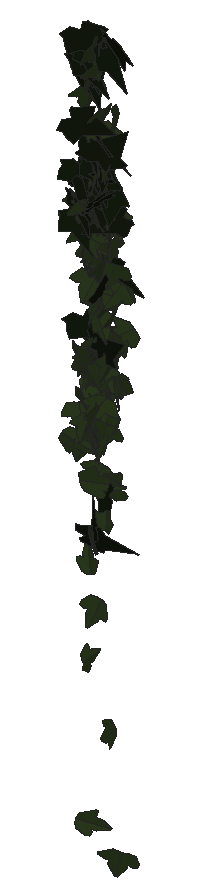
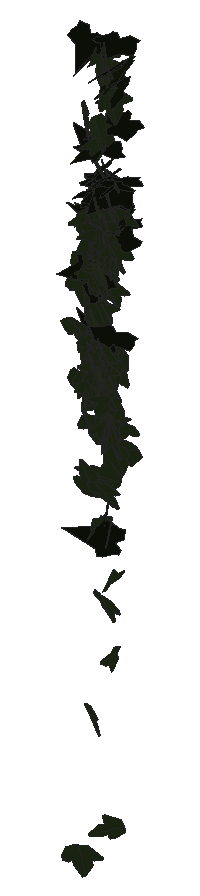
# SketchUp Ruby script. Lengths in inches.
U = 1.inch
M = Sketchup.active_model
def pt(a) = Geom::Point3d.new(a.map { |v| v * U })
def face(e, loops, mat)
  f = e.add_face(loops[0].map { |a| pt(a) })
  loops[1..].each { |l| e.add_face(l.map { |a| pt(a) }).erase! }
  f.material = f.back_material = mat if mat
  f
end
# faces: each face lists its corners as indices into pts; further lists are holes
def faces(e, pts, list, mat = nil) = list.each { |f| face(e, (f[0].is_a?(Array) ? f : [f]).map { |l| l.map { |i| pts[i] } }, mat) }
# xy, xz, yz: faces in a plane at the given z, y or x. An outline is a flat list of corners, or four numbers for a rectangle; further outlines are holes
def ring(l) = l.size == 4 ? [[l[0], l[1]], [l[2], l[1]], [l[2], l[3]], [l[0], l[3]]] : l.each_slice(2).to_a
def flat(e, list, mat, &to3) = list.each { |f| face(e, (f[0].is_a?(Array) ? f : [f]).map { |l| ring(l).map { |u, v| to3.(u, v) } }, mat) }
def xy(e, z, list, mat = nil) = flat(e, list, mat) { |x, y| [x, y, z] }
def xz(e, y, list, mat = nil) = flat(e, list, mat) { |x, z| [x, y, z] }
def yz(e, x, list, mat = nil) = flat(e, list, mat) { |y, z| [x, y, z] }
def lines(e, pts, list) = list.each { |a, b| e.add_line(pt(pts[a]), pt(pts[b])) }
# prism: a flat outline (further loops are holes) pulled along v
def prism(e, loops, v, mat = nil)
  f = face(e, loops, mat); d = Geom::Vector3d.new(v.map { |x| x * U })
  f.pushpull(f.normal.samedirection?(d) ? d.length : -d.length)
end
def box(e, o, s, mat = nil) = prism(e, [[o, [o[0] + s[0], o[1], o[2]], [o[0] + s[0], o[1] + s[1], o[2]], [o[0], o[1] + s[1], o[2]]]], [0, 0, s[2]], mat)
def at(x, y, z, deg = 0) = Geom::Transformation.translation(pt([x, y, z])) * Geom::Transformation.rotation(ORIGIN, Z_AXIS, deg.degrees)
def axes(o, x, y, z) = Geom::Transformation.new([*x, 0, *y, 0, *z, 0, *pt(o).to_a, 1])
def part(name) = M.definitions.add(name)
# library, detail: a bought-in or finely detailed component or shape, given as its bounding box
def library(name, o, s) = part(name).tap { |d| box(d.entities, o, s) }
def detail(e, o, s) = box(e.add_group.entities, o, s)
def put(e, d, t, mat = nil) = e.add_instance(d, t).tap { |i| i.material = mat if mat }
def group(e, t, mat = nil) = e.add_group.tap { |g| g.transformation = t; g.material = mat if mat }.entities
root = M.entities
M.materials.add("1026 AP 7946 SUNNY SIDE UP").color = [254, 231, 186]
M.materials.add("efeu1").color = [18, 25, 13]
M.materials.add("efeu2").color = [43, 57, 29]
c1 = part("ivyleaf_10")
p = [[0,0.5,-0.03],[-0.0625,2.02,-0.43],[-0.19,2.01,-0.46],[-0.54,1.05,-0.29],[-0.52,0.625,-0.18],[-0.83,0.76,-0.28],
  [-1.16,0.64,-0.33],[-1.15,0.33,-0.24],[-0.77,-0.39,0.02],[-0.3,-0.51,0.16],[0.04,-0.48,0.23],[-0.02,2.01,-0.4375],
  [-0.06,2.01,-0.43],[0.04,-0.49,0.23],[0.67,-0.49,0.14],[1.38,0.36,-0.2],[1.375,0.51,-0.24],[0.81,0.65,-0.19],
  [0.62,0.59,-0.15],[0.6,1.09,-0.28],[0.5,1.23,-0.31]]
faces(c1.entities,p,[[0,1,2,3,4,5,6,7,8,9,10],[11,12,0,13,14,15,16,17,18,19,20]],"efeu2")
c2 = part("ivyleaf_9")
p = [[1.54,2.16,1.25],[1.36,2.04,1.19],[-0.21,0.99,0.68],[-0.71,1.11,0.82],[-0.85,0.86,0.67],[-0.8,0.17,0.21],
  [-0.9,-0.01,0.1],[-0.67,-0.16,-0.02],[-0.08,-0.08,-0.05],[-0.03,-0.6,-0.4],[0.65,-0.88,-0.66],[0.83,-0.6,-0.49],
  [1.29,-0.42,-0.43],[1.8125,-0.07,-0.26],[1.21,0.44,0.15]]
faces(c2.entities,p,[[0,1,2,3,4,5,6,7,8,9,10,11,12,13,14]],"efeu1")
put(root,c1,axes([108.3,212.91,255.9375],[0.03585,0.20195,-0.10025],[-0.01427,0.09971,0.20911],[0.35299,-0.01648,0.01864]),"1026 AP 7946 SUNNY SIDE UP")
put(root,c1,axes([108.32,212.78,258.74],[-0.16539,-0.18433,0.05734],[-0.02204,-0.05711,-0.21838],[0.30245,-0.10496,0.01544]),"1026 AP 7946 SUNNY SIDE UP")
put(root,c1,axes([108.23,212.85,263.3125],[-0.15686,-0.19603,-0.08454],[0.10648,0.05533,-0.22369],[0.31603,-0.11594,0.03341]),"1026 AP 7946 SUNNY SIDE UP")
put(root,c1,axes([108.16,212.79,259.41],[0.32743,0.06448,0.04041],[0.06834,-0.00965,-0.22351],[-0.09666,0.21161,-0.02115]),"1026 AP 7946 SUNNY SIDE UP")
put(root,c2,axes([108.09,212.86,267.29],[0.11956,-0.23605,0.07715],[0.01461,-0.07697,-0.25552],[0.38977,0.07529,-0.01409]),"1026 AP 7946 SUNNY SIDE UP")
put(root,c1,axes([108.23,212.96,259.5],[0.20788,-0.1548,0.06197],[0.06128,-0.04698,-0.20999],[0.25437,0.13782,-0.00005]),"1026 AP 7946 SUNNY SIDE UP")
put(root,c1,axes([108.29,212.83,264.08],[-0.31893,-0.13051,-0.03285],[0.0708,-0.01303,-0.24591],[0.19874,-0.20479,0.03489]),"1026 AP 7946 SUNNY SIDE UP")
put(root,c2,axes([108.3,212.76,263.42],[0.3299,-0.04343,0.14661],[-0.19696,0.08199,0.21612],[-0.12697,-0.24004,0.04568]),"1026 AP 7946 SUNNY SIDE UP")
put(root,c2,axes([108.13,212.78,263.96],[0.09045,-0.22029,0.08276],[0.01722,-0.08139,-0.23483],[0.36898,0.0578,-0.00933]),"1026 AP 7946 SUNNY SIDE UP")
put(root,c1,axes([108.06,212.63,258.83],[-0.13369,-0.02534,-0.21212],[0.32396,-0.03512,-0.08345],[-0.03634,-0.21985,0.03644]),"1026 AP 7946 SUNNY SIDE UP")
put(root,c1,axes([108.35,212.89,260.68],[-0.08695,-0.2082,0.03204],[0.00749,-0.03461,-0.2217],[0.3312,-0.05388,0.01343]),"1026 AP 7946 SUNNY SIDE UP")
put(root,c1,axes([108.4375,212.6,262.91],[-0.13162,0.14112,0.18624],[-0.19898,0.13107,-0.16573],[-0.29956,-0.14907,0.02825]),"1026 AP 7946 SUNNY SIDE UP")
put(root,c1,axes([108.27,212.79,259.75],[-0.27149,0.10699,-0.06247],[0.06175,-0.05217,-0.20826],[-0.18375,-0.17561,0.02231]),"1026 AP 7946 SUNNY SIDE UP")
put(root,c1,axes([108.32,212.6,260.83],[-0.27688,0.12701,-0.02084],[0.01369,-0.02366,-0.22333],[-0.20194,-0.17574,0.01343]),"1026 AP 7946 SUNNY SIDE UP")
put(root,c1,axes([108.37,212.88,264.01],[-0.10025,-0.20706,0.10917],[0.01574,-0.11341,-0.22031],[0.36626,-0.0518,0.03935]),"1026 AP 7946 SUNNY SIDE UP")
put(root,c1,axes([108.36,212.91,264.375],[0.16184,-0.22019,-0.00198],[0.0034,0.00175,-0.25037],[0.34622,0.10291,0.00338]),"1026 AP 7946 SUNNY SIDE UP")
put(root,c1,axes([108.33,212.96,260.63],[-0.09556,0.20553,-0.00679],[-0.01012,-0.00999,-0.22066],[-0.32324,-0.06044,0.00892]),"1026 AP 7946 SUNNY SIDE UP")
put(root,c2,axes([108.14,212.78,264.02],[0.25616,-0.16725,0.06236],[0.04924,-0.05513,-0.24031],[0.27582,0.16516,-0.01501]),"1026 AP 7946 SUNNY SIDE UP")
put(root,c1,axes([108.375,212.65,264.04],[-0.05121,-0.24291,0.00007],[0.06408,-0.0069,-0.24891],[0.37654,-0.03186,0.04237]),"1026 AP 7946 SUNNY SIDE UP")
put(root,c2,axes([108.26,212.61,263.75],[-0.01152,-0.22482,-0.10831],[0.01323,0.10362,-0.23108],[0.38919,-0.01018,0.00465]),"1026 AP 7946 SUNNY SIDE UP")
put(root,c1,axes([108.43,212.75,260.69],[-0.00835,-0.21864,0.06836],[-0.0072,-0.06751,-0.22568],[0.35978,-0.00642,-0.00293]),"1026 AP 7946 SUNNY SIDE UP")
put(root,c1,axes([108.33,212.94,260.41],[0.14731,-0.19752,0.00171],[0.00528,0.00467,0.22518],[-0.31057,-0.09361,0.00464]),"1026 AP 7946 SUNNY SIDE UP")
put(root,c1,axes([108.47,213.0625,258.05],[0.30017,-0.04016,-0.09755],[-0.15281,-0.00651,-0.19951],[0.05195,0.21289,-0.02321]),"1026 AP 7946 SUNNY SIDE UP")
put(root,c2,axes([108.28,212.71,264.79],[-0.10135,-0.21014,-0.11428],[0.08548,0.09758,-0.22484],[0.36282,-0.08169,0.02105]),"1026 AP 7946 SUNNY SIDE UP")
put(root,c2,axes([108.2,212.74,266.79],[0.25123,-0.19863,0.00638],[-0.01575,-0.01742,-0.26201],[0.31215,0.15899,-0.01835]),"1026 AP 7946 SUNNY SIDE UP")
put(root,c1,axes([108.3,212.99,260],[0.17595,0.16302,0.0853],[0.07141,0.06814,-0.2033],[-0.27782,0.12076,0.00177]),"1026 AP 7946 SUNNY SIDE UP")
put(root,c1,axes([108.47,212.74,266.57],[-0.13179,-0.24609,0.01208],[0.00255,-0.01441,-0.26783],[0.3875,-0.0836,0.00587]),"1026 AP 7946 SUNNY SIDE UP")
put(root,c1,axes([108.44,212.75,259.19],[-0.02132,-0.12753,-0.18169],[0.02214,0.1751,-0.13107],[0.34059,-0.01937,-0.00285]),"1026 AP 7946 SUNNY SIDE UP")
put(root,c1,axes([108.41,212.8125,260.29],[0.21781,-0.1573,0.04926],[0.03174,-0.04696,-0.21561],[0.25698,0.13913,-0.01513]),"1026 AP 7946 SUNNY SIDE UP")
put(root,c1,axes([108.54,212.72,259.07],[0.21736,-0.11788,-0.14784],[-0.15263,0.10568,-0.186],[0.248,0.16835,0.0151]),"1026 AP 7946 SUNNY SIDE UP")
put(root,c1,axes([108.67,212.6,263.12],[-0.18064,0.08381,0.19989],[-0.31223,0.03135,-0.13522],[-0.11184,-0.22289,0.05463]),"1026 AP 7946 SUNNY SIDE UP")
put(root,c1,axes([108.4375,212.69,259.31],[-0.08917,-0.1936,0.09796],[0.06133,-0.10697,-0.19874],[0.33434,-0.03201,0.06258]),"1026 AP 7946 SUNNY SIDE UP")
put(root,c2,axes([108.29,212.45,265.97],[0.09508,-0.02675,-0.26595],[-0.00984,0.2647,-0.02823],[0.40775,0.01263,0.06133]),"1026 AP 7946 SUNNY SIDE UP")
put(root,c1,axes([108.48,213.01,260.63],[0.05744,-0.20837,0.04319],[-0.00152,-0.0439,-0.21802],[0.33458,0.03557,-0.00841]),"1026 AP 7946 SUNNY SIDE UP")
put(root,c1,axes([108.375,212.83,264.06],[-0.24999,0.12324,-0.13135],[0.09783,-0.12255,-0.20157],[-0.26195,-0.16338,0.05008]),"1026 AP 7946 SUNNY SIDE UP")
put(root,c1,axes([108.43,212.91,263.41],[0.2434,-0.17927,0.01394],[0.03051,-0.00244,-0.24365],[0.28116,0.15546,0.01437]),"1026 AP 7946 SUNNY SIDE UP")
put(root,c1,axes([108.31,212.75,250.43],[0.06067,0.05904,0.21124],[0.14435,0.18313,-0.07116],[-0.30231,0.09929,0.00841]),"1026 AP 7946 SUNNY SIDE UP")
put(root,c1,axes([108.53,212.94,260.67],[0.30924,-0.04393,-0.07935],[-0.1162,0.02126,-0.20743],[0.07644,0.21005,0.0057]),"1026 AP 7946 SUNNY SIDE UP")
put(root,c2,axes([108.35,212.625,267.83],[-0.0154,-0.13388,-0.23906],[0.0172,0.23105,-0.1369],[0.41986,-0.01437,-0.00316]),"1026 AP 7946 SUNNY SIDE UP")
put(root,c1,axes([108.51,212.92,262.78],[0.0284,-0.23227,0.00314],[0.00325,-0.00422,-0.24002],[0.36527,0.01809,0.00189]),"1026 AP 7946 SUNNY SIDE UP")
put(root,c2,axes([108.29,212.82,261.42],[-0.04734,-0.13054,-0.23252],[0.14938,0.2053,-0.13463],[0.38073,-0.09679,0.02391]),"1026 AP 7946 SUNNY SIDE UP")
put(root,c2,axes([108.35,212.68,264.58],[0.33632,0.13585,0.03196],[0.05542,0.00079,-0.26037],[-0.21171,0.21602,-0.01739]),"1026 AP 7946 SUNNY SIDE UP")
put(root,c1,axes([108.43,212.68,260.49],[-0.32432,0.00476,-0.076],[0.11491,-0.02037,-0.21189],[-0.0178,-0.21811,0.01684]),"1026 AP 7946 SUNNY SIDE UP")
put(root,c1,axes([108.68,212.89,260.05],[0.11551,-0.0324,-0.20546],[-0.25531,0.11651,-0.0805],[0.18861,0.17755,0.01685]),"1026 AP 7946 SUNNY SIDE UP")
put(root,c1,axes([108.43,212.86,263.16],[-0.19912,0.16735,-0.10418],[0.07102,-0.09334,-0.21592],[-0.29993,-0.13321,0.01803]),"1026 AP 7946 SUNNY SIDE UP")
put(root,c1,axes([108.5,213.01,260.56],[0.1894,0.16173,-0.07732],[-0.06136,-0.06561,-0.20799],[-0.27419,0.1264,-0.00687]),"1026 AP 7946 SUNNY SIDE UP")
put(root,c1,axes([108.51,212.78,262.4],[0.3797,0.01554,-0.03948],[-0.05786,-0.02397,-0.24846],[-0.02996,0.24334,-0.02051]),"1026 AP 7946 SUNNY SIDE UP")
put(root,c1,axes([108.49,212.57,254.11],[0.0272,0.00065,-0.22081],[0.07127,0.21016,0.00565],[0.32941,-0.04553,0.01701]),"1026 AP 7946 SUNNY SIDE UP")
put(root,c2,axes([108.32,212.63,267.25],[0.1657,-0.22923,-0.06433],[0.01618,0.07126,-0.25652],[0.37269,0.09882,0.03974]),"1026 AP 7946 SUNNY SIDE UP")
put(root,c2,axes([108.37,212.84,266.88],[0.05154,-0.23925,0.08434],[0.03022,-0.08133,-0.24913],[0.39716,0.03724,0.00801]),"1026 AP 7946 SUNNY SIDE UP")
put(root,c2,axes([108.41,212.9,267.24],[-0.00476,-0.25563,0.02473],[0.00016,-0.02546,-0.26352],[0.40394,-0.003,0.0004]),"1026 AP 7946 SUNNY SIDE UP")
put(root,c2,axes([108.41,212.65,264.5625],[0.1257,-0.18876,-0.13545],[-0.06552,0.12386,-0.21028],[0.35476,0.08976,0.00916]),"1026 AP 7946 SUNNY SIDE UP")
put(root,c1,axes([108.56,212.9,262.88],[0.06698,-0.22885,0.03069],[0.00245,-0.03133,-0.23995],[0.36314,0.04242,-0.00405]),"1026 AP 7946 SUNNY SIDE UP")
put(root,c1,axes([108.61,212.66,259.15],[-0.18403,0.17134,0.09845],[-0.11454,0.06416,-0.2122],[-0.28563,-0.13612,0.02166]),"1026 AP 7946 SUNNY SIDE UP")
put(root,c1,axes([108.53,212.95,261.08],[0.1876,-0.18526,0.0281],[0.02929,-0.02169,-0.2271],[0.29323,0.12069,0.00471]),"1026 AP 7946 SUNNY SIDE UP")
put(root,c1,axes([108.6,212.89,260.99],[-0.34279,0.03021,0.00648],[-0.01793,-0.0384,-0.22326],[-0.04504,-0.21468,0.03953]),"1026 AP 7946 SUNNY SIDE UP")
put(root,c1,axes([108.65,212.91,261.89],[-0.19044,-0.17871,0.07467],[-0.03561,-0.07301,-0.22178],[0.30175,-0.12141,0.02095]),"1026 AP 7946 SUNNY SIDE UP")
put(root,c1,axes([108.46,212.76,259.8],[0.08285,0.05796,-0.20445],[0.17099,0.16682,0.08078],[0.27708,-0.12027,0.01129]),"1026 AP 7946 SUNNY SIDE UP")
put(root,c1,axes([108.3125,212.98,263.98],[0.19181,0.00767,0.20816],[0.31788,-0.00306,-0.12565],[-0.00211,0.23597,-0.00702]),"1026 AP 7946 SUNNY SIDE UP")
put(root,c1,axes([108.53,212.83,259.34],[0.0392,0.21212,-0.01266],[0.00229,-0.01376,-0.22009],[-0.33421,0.02479,-0.00299]),"1026 AP 7946 SUNNY SIDE UP")
put(root,c1,axes([108.53,212.93,264.1],[0.16128,-0.19924,0.08512],[0.08377,-0.06654,-0.23067],[0.32935,0.11449,0.01699]),"1026 AP 7946 SUNNY SIDE UP")
put(root,c1,axes([108.57,212.79,263.98],[0.10939,-0.21804,-0.08029],[0.04222,0.08718,-0.22972],[0.36098,0.05588,0.0512]),"1026 AP 7946 SUNNY SIDE UP")
put(root,c2,axes([108.56,212.87,264.7],[-0.27246,-0.18028,-0.06789],[0.09114,0.03406,-0.25676],[0.28716,-0.18186,0.01707]),"1026 AP 7946 SUNNY SIDE UP")
put(root,c1,axes([108.625,212.96,266.02],[-0.0196,-0.24747,-0.00193],[0.0003,0.00046,-0.25526],[0.38912,-0.01246,0.0001]),"1026 AP 7946 SUNNY SIDE UP")
put(root,c1,axes([108.6875,212.66,262.99],[0.12873,-0.14201,-0.17334],[-0.11618,0.15048,-0.16779],[0.3251,0.11,0.00867]),"1026 AP 7946 SUNNY SIDE UP")
put(root,c1,axes([108.63,212.91,261.04],[-0.16633,-0.198,-0.00073],[0.01765,-0.00647,-0.23092],[0.31084,-0.10558,0.01272]),"1026 AP 7946 SUNNY SIDE UP")
put(root,c1,axes([108.55,212.95,260.29],[-0.15362,0.18463,-0.04774],[0.02826,-0.04409,-0.2154],[-0.29839,-0.09923,0.00418]),"1026 AP 7946 SUNNY SIDE UP")
put(root,c1,axes([108.53,213.01,260.68],[0.20278,0.16344,0.06108],[0.00763,0.06929,-0.21053],[-0.27278,0.12344,0.03952]),"1026 AP 7946 SUNNY SIDE UP")
put(root,c1,axes([108.62,212.6,267.58],[-0.00349,-0.22215,-0.13505],[0.0365,0.12913,-0.22729],[0.40294,-0.01362,0.01942]),"1026 AP 7946 SUNNY SIDE UP")
put(root,c1,axes([108.67,212.94,262.72],[-0.31337,-0.11322,0.02178],[-0.01434,-0.02788,-0.23543],[0.18073,-0.19853,0.01908]),"1026 AP 7946 SUNNY SIDE UP")
put(root,c1,axes([108.7,212.79,267.49],[-0.06676,0.24723,0.07404],[-0.15584,0.05016,-0.24252],[-0.37298,-0.06521,0.08808]),"1026 AP 7946 SUNNY SIDE UP")
put(root,c1,axes([108.56,212.96,263.59],[0.23631,0.17998,-0.01623],[0.00093,-0.0223,-0.24121],[-0.28422,0.14957,-0.01428]),"1026 AP 7946 SUNNY SIDE UP")
put(root,c1,axes([108.64,213,260.75],[0.04838,-0.18821,0.10508],[0.01552,-0.10277,-0.19697],[0.33706,0.03175,-0.00601]),"1026 AP 7946 SUNNY SIDE UP")
put(root,c1,axes([108.52,212.74,264.83],[0.25786,-0.12979,0.11872],[0.1292,-0.08274,-0.21558],[0.24127,0.18303,-0.01144]),"1026 AP 7946 SUNNY SIDE UP")
put(root,c1,axes([108.65,212.88,264.24],[0.08162,-0.2357,0.02709],[0.00396,-0.02774,-0.24877],[0.37314,0.05185,-0.00329]),"1026 AP 7946 SUNNY SIDE UP")
put(root,c1,axes([108.56,212.92,265.63],[0.14973,0.23947,-0.00839],[0.00778,-0.01219,-0.26539],[-0.37676,0.09492,-0.00882]),"1026 AP 7946 SUNNY SIDE UP")
put(root,c2,axes([108.5,212.87,264.8125],[0.04109,-0.24429,-0.01123],[-0.00149,0.00947,-0.25305],[0.38442,0.02615,0.00022]),"1026 AP 7946 SUNNY SIDE UP")
put(root,c1,axes([108.69,212.5,256.92],[-0.1859,0.17647,0.08299],[-0.09035,0.05703,-0.21795],[-0.29066,-0.1306,0.01467]),"1026 AP 7946 SUNNY SIDE UP")
put(root,c1,axes([108.73,212.94,262.59],[0.25146,-0.18799,-0.08283],[-0.10887,0.04482,-0.25294],[0.30181,0.1728,-0.02223]),"1026 AP 7946 SUNNY SIDE UP")
put(root,c1,axes([108.63,212.77,261.93],[0.18825,-0.18257,0.07134],[0.03688,-0.06842,-0.22463],[0.30539,0.1208,-0.01685]),"1026 AP 7946 SUNNY SIDE UP")
put(root,c1,axes([108.7,212.66,267.09],[-0.00228,-0.24958,0.06638],[-0.00904,-0.06581,-0.25745],[0.40577,-0.00287,-0.00536]),"1026 AP 7946 SUNNY SIDE UP")
put(root,c1,axes([108.69,212.9,262.875],[0.06635,-0.23047,0.01305],[0.00117,-0.01407,-0.24145],[0.36306,0.04216,-0.00161]),"1026 AP 7946 SUNNY SIDE UP")
put(root,c1,axes([108.68,212.68,259.64],[0.03796,-0.22006,0.05305],[0.01014,-0.05236,-0.22837],[0.35568,0.02498,0.00085]),"1026 AP 7946 SUNNY SIDE UP")
put(root,c1,axes([108.56,212.95,260.91],[-0.24543,0.07322,-0.1393],[0.13398,-0.11987,-0.16838],[-0.20197,-0.1685,0.05758]),"1026 AP 7946 SUNNY SIDE UP")
put(root,c1,axes([108.74,212.78,259.75],[0.22523,0.10862,-0.12048],[-0.15739,-0.06233,-0.18532],[-0.1964,0.17451,0.01034]),"1026 AP 7946 SUNNY SIDE UP")
put(root,c1,axes([108.71,212.88,257.02],[0.03339,0.15549,-0.15441],[-0.00127,0.15155,0.16179],[0.34056,-0.01468,0.01574]),"1026 AP 7946 SUNNY SIDE UP")
put(root,c1,axes([108.67,212.59,258.96],[-0.12907,0.20428,0.00536],[-0.01458,0.00063,-0.22663],[-0.32094,-0.08218,0.00814]),"1026 AP 7946 SUNNY SIDE UP")
put(root,c1,axes([108.68,212.6875,255.33],[0.33005,-0.11593,-0.00269],[-0.01827,-0.017,-0.24623],[0.1814,0.20922,-0.0199]),"1026 AP 7946 SUNNY SIDE UP")
put(root,c1,axes([108.69,212.68,267.2],[0.26622,-0.19457,0.01336],[-0.00617,-0.02202,-0.26524],[0.30669,0.16846,-0.01693]),"1026 AP 7946 SUNNY SIDE UP")
put(root,c2,axes([108.76,212.54,257],[-0.008,-0.11114,0.22877],[0.06676,0.21909,0.11493],[-0.38562,0.04023,0.01515]),"1026 AP 7946 SUNNY SIDE UP")
put(root,c2,axes([108.58,212.95,264.9375],[0.00269,-0.21254,0.11753],[-0.00111,-0.1153,-0.21963],[0.3802,0.00117,-0.00147]),"1026 AP 7946 SUNNY SIDE UP")
put(root,c1,axes([108.61,212.95,263.64],[0.3599,0.04608,0.03053],[0.04937,-0.00738,-0.24018],[-0.07033,0.23065,-0.01237]),"1026 AP 7946 SUNNY SIDE UP")
put(root,c1,axes([108.65,212.93,262.69],[0.30505,0.12305,-0.01256],[-0.00393,-0.02006,-0.23624],[-0.19451,0.19339,-0.01492]),"1026 AP 7946 SUNNY SIDE UP")
put(root,c1,axes([108.75,212.97,260.69],[0.17246,-0.1823,-0.04853],[-0.03667,0.03973,-0.21894],[0.29338,0.11213,0.00116]),"1026 AP 7946 SUNNY SIDE UP")
put(root,c1,axes([108.54,212.92,260.28],[0.11313,-0.08592,0.18658],[0.26455,-0.07965,-0.10796],[0.17264,0.17836,0.04317]),"1026 AP 7946 SUNNY SIDE UP")
put(root,c1,axes([108.75,212.95,260.17],[-0.2459,-0.1487,-0.01899],[0.06069,-0.01546,-0.21899],[0.22749,-0.15661,0.0379]),"1026 AP 7946 SUNNY SIDE UP")
put(root,c1,axes([108.76,212.99,261.125],[0.03262,0.17122,0.14253],[-0.0743,0.13824,-0.16933],[-0.33709,-0.0139,0.05112]),"1026 AP 7946 SUNNY SIDE UP")
put(root,c1,axes([108.76,212.89,261.8],[0.07673,-0.21593,0.04833],[0.01734,-0.04686,-0.22834],[0.34744,0.05003,0.00072]),"1026 AP 7946 SUNNY SIDE UP")
put(root,c1,axes([108.66,212.79,260.48],[-0.29635,-0.03959,-0.10134],[0.16634,-0.07603,-0.17813],[-0.00461,-0.19843,0.0871]),"1026 AP 7946 SUNNY SIDE UP")
put(root,c2,axes([108.42,212.73,256.72],[0.23941,-0.03397,0.20907],[0.30423,-0.063,-0.16062],[0.111,0.24592,-0.0107]),"1026 AP 7946 SUNNY SIDE UP")
put(root,c1,axes([108.72,212.625,263.35],[-0.00815,0.17711,0.17325],[0.00015,0.16721,-0.18152],[-0.38294,-0.0037,-0.00376]),"1026 AP 7946 SUNNY SIDE UP")
put(root,c1,axes([108.86,212.76,259.24],[-0.32637,-0.02516,0.04859],[-0.06584,-0.0419,-0.21248],[0.05255,-0.20872,0.03551]),"1026 AP 7946 SUNNY SIDE UP")
put(root,c2,axes([108.7,212.4375,264.1875],[0.13478,0.09086,0.2155],[0.15741,0.18519,-0.12435],[-0.32138,0.12881,0.02946]),"1026 AP 7946 SUNNY SIDE UP")
put(root,c2,axes([108.66,212.87,264.1],[-0.06257,-0.20151,0.13204],[0.04925,-0.13434,-0.20652],[0.37325,-0.01605,0.04938]),"1026 AP 7946 SUNNY SIDE UP")
put(root,c2,axes([109.03,212.6,257.91],[-0.1133,0.00417,-0.23727],[-0.35365,0.051,0.07373],[0.07846,0.2359,-0.0103]),"1026 AP 7946 SUNNY SIDE UP")
put(root,c1,axes([108.83,212.96,261.16],[-0.12735,-0.20362,0.03169],[0.00588,-0.03574,-0.22532],[0.32402,-0.07938,0.01654]),"1026 AP 7946 SUNNY SIDE UP")
put(root,c1,axes([108.8125,212.86,263.49],[0.15606,-0.15988,-0.15235],[-0.00923,0.15957,-0.18196],[0.34136,0.07741,0.06473]),"1026 AP 7946 SUNNY SIDE UP")
put(root,c2,axes([108.73,212.73,262.11],[0.13531,0.16069,0.17207],[-0.14833,-0.13739,0.18647],[0.33176,-0.12697,0.0132]),"1026 AP 7946 SUNNY SIDE UP")
put(root,c1,axes([108.8,212.96,260.96],[0.10372,-0.20406,0.04736],[0.02002,-0.04541,-0.22119],[0.32871,0.06715,-0.00147]),"1026 AP 7946 SUNNY SIDE UP")
put(root,c1,axes([108.55,212.61,258.02],[-0.06861,-0.00382,0.25168],[0.32356,0.13329,0.04078],[-0.20723,0.20937,-0.01965]),"1026 AP 7946 SUNNY SIDE UP")
put(root,c1,axes([108.78,213.12,260],[-0.14706,0.17053,-0.08989],[0.03118,-0.08903,-0.19946],[-0.30029,-0.09276,0.02331]),"1026 AP 7946 SUNNY SIDE UP")
put(root,c1,axes([108.85,212.66,264.55],[0.02097,-0.22304,-0.13461],[0.02424,0.13003,-0.22849],[0.40473,0.00377,0.02066]),"1026 AP 7946 SUNNY SIDE UP")
put(root,c2,axes([108.65,212.84,265.48],[0.29997,-0.15506,-0.04586],[-0.04853,0.03119,-0.25303],[0.24859,0.1932,0.00594]),"1026 AP 7946 SUNNY SIDE UP")
put(root,c1,axes([108.78,212.64,261.68],[0.04326,0.23277,0.01026],[0.00952,0.00798,-0.24136],[-0.36614,0.02771,-0.00506]),"1026 AP 7946 SUNNY SIDE UP")
put(root,c1,axes([108.91,212.86,263.89],[0.13729,0.19804,-0.09928],[-0.16718,-0.05416,-0.21173],[-0.30418,0.11915,0.07155]),"1026 AP 7946 SUNNY SIDE UP")
put(root,c1,axes([108.86,212.71,265.01],[0.22723,-0.19943,0.02508],[0.00546,-0.02889,-0.25347],[0.31608,0.14387,-0.01365]),"1026 AP 7946 SUNNY SIDE UP")
put(root,c1,axes([108.89,212.6,262.94],[0.00764,-0.23574,-0.03977],[0.00876,0.03738,-0.24261],[0.37518,0.00393,0.00648]),"1026 AP 7946 SUNNY SIDE UP")
put(root,c2,axes([108.82,212.45,264.26],[0.14489,0.14391,0.18086],[0.11193,0.16067,-0.17405],[-0.33788,0.11493,0.0199]),"1026 AP 7946 SUNNY SIDE UP")
put(root,c1,axes([108.79,212.875,257.83],[-0.37699,-0.00091,0.10145],[0.15386,0.02726,0.24582],[-0.01759,0.25775,-0.02411]),"1026 AP 7946 SUNNY SIDE UP")
put(root,c1,axes([108.88,212.85,263.23],[-0.12379,-0.21371,-0.06168],[0.06105,0.04799,-0.23351],[0.34308,-0.08565,0.0193]),"1026 AP 7946 SUNNY SIDE UP")
put(root,c1,axes([108.88,212.66,258.99],[0.1939,-0.17443,0.01769],[0.00115,-0.02169,-0.21985],[0.27576,0.12274,-0.01152]),"1026 AP 7946 SUNNY SIDE UP")
put(root,c1,axes([109.07,212.95,260.09],[-0.27451,-0.0053,-0.1316],[-0.20043,0.02328,0.17865],[0.01493,0.21505,-0.02131]),"1026 AP 7946 SUNNY SIDE UP")
put(root,c1,axes([108.93,212.86,261.72],[0.06532,-0.21852,-0.04391],[-0.01549,0.04025,-0.2289],[0.34936,0.04264,-0.00194]),"1026 AP 7946 SUNNY SIDE UP")
put(root,c2,axes([108.61,212.92,262.71],[0.01253,-0.02704,-0.26463],[0.33773,0.14318,-0.00783],[0.22517,-0.21324,0.02647]),"1026 AP 7946 SUNNY SIDE UP")
put(root,c2,axes([108.77,212.625,265.18],[-0.21635,0.03595,0.21779],[0.32902,-0.03132,0.14574],[0.0723,0.25011,-0.01154]),"1026 AP 7946 SUNNY SIDE UP")
put(root,c2,axes([108.69,212.7,260.92],[-0.04359,0.03495,0.25587],[0.22122,-0.20447,0.04466],[0.32614,0.14336,0.0039]),"1026 AP 7946 SUNNY SIDE UP")
put(root,c1,axes([108.9375,212.79,260.76],[-0.04556,-0.20542,0.10624],[0.02428,-0.10661,-0.21252],[0.36143,-0.01873,0.02767]),"1026 AP 7946 SUNNY SIDE UP")
put(root,c1,axes([109.01,213.03,249.77],[-0.3157,-0.10423,0.04945],[-0.05293,-0.04022,-0.23239],[0.17291,-0.20262,0.01915]),"1026 AP 7946 SUNNY SIDE UP")
put(root,c2,axes([108.86,212.88,264.43],[-0.0782,-0.23661,0.03136],[0.00269,-0.03282,-0.24912],[0.37537,-0.04905,0.00832]),"1026 AP 7946 SUNNY SIDE UP")
put(root,c2,axes([108.8,212.79,267.46],[0.15924,-0.22492,-0.10067],[-0.07561,0.08405,-0.25346],[0.3773,0.11177,-0.0083]),"1026 AP 7946 SUNNY SIDE UP")
put(root,c2,axes([109.14,212.85,263.93],[-0.37621,0.00045,0.03349],[-0.05095,-0.02292,-0.2455],[0.00415,-0.24036,0.02205]),"1026 AP 7946 SUNNY SIDE UP")
put(root,c1,axes([109.07,212.86,262.33],[-0.32855,-0.03884,0.0955],[-0.09613,-0.12117,-0.19449],[0.12586,-0.19394,0.10077]),"1026 AP 7946 SUNNY SIDE UP")
put(root,c1,axes([108.99,212.86,261.22],[-0.26838,0.14192,-0.00108],[-0.04791,-0.03947,-0.22307],[-0.21797,-0.16607,0.05036]),"1026 AP 7946 SUNNY SIDE UP")
put(root,c1,axes([108.97,212.88,259.38],[0.20292,-0.17121,0.02378],[0.00612,-0.02714,-0.22061],[0.27179,0.12844,-0.01279]),"1026 AP 7946 SUNNY SIDE UP")
put(root,c1,axes([109.06,212.93,262.35],[-0.34252,0.05726,0.05472],[-0.09651,-0.02971,-0.2279],[-0.07537,-0.22216,0.04317]),"1026 AP 7946 SUNNY SIDE UP")
put(root,c1,axes([108.97,212.96,261.18],[0.19211,-0.18458,-0.02035],[0.01027,0.02666,-0.22693],[0.29154,0.12069,0.0214]),"1026 AP 7946 SUNNY SIDE UP")
put(root,c1,axes([108.93,212.91,263.85],[0.07297,0.23579,0.0021],[-0.01037,0.00201,-0.24746],[-0.37062,0.04637,0.00734]),"1026 AP 7946 SUNNY SIDE UP")
put(root,c1,axes([109.06,212.65,252.72],[0.1745,-0.15402,-0.11389],[-0.10138,0.08873,-0.19505],[0.27949,0.12834,0.00035]),"1026 AP 7946 SUNNY SIDE UP")
put(root,c1,axes([109.07,212.72,262.83],[-0.29251,-0.12159,0.0551],[-0.04771,-0.05192,-0.22767],[0.2038,-0.18667,0.02579]),"1026 AP 7946 SUNNY SIDE UP")
put(root,c1,axes([109.02,212.96,261.11],[0.273,-0.12814,-0.02936],[-0.05505,-0.0009,-0.22122],[0.19869,0.17582,-0.02095]),"1026 AP 7946 SUNNY SIDE UP")
put(root,c1,axes([108.97,212.88,260.27],[-0.12681,-0.19151,-0.06254],[0.08676,0.0406,-0.211],[0.30323,-0.09171,0.03421]),"1026 AP 7946 SUNNY SIDE UP")
put(root,c2,axes([108.97,212.77,267.77],[0.34765,-0.03488,-0.15721],[-0.23954,0.01129,-0.23027],[0.05528,0.26829,-0.00915]),"1026 AP 7946 SUNNY SIDE UP")
put(root,c1,axes([109.04,212.82,266.11],[0.16328,-0.21793,-0.08709],[-0.01732,0.0865,-0.24677],[0.36645,0.10119,0.02714]),"1026 AP 7946 SUNNY SIDE UP")
put(root,c1,axes([109.22,213,261.39],[-0.2474,0.06703,0.14097],[-0.23844,-0.08323,-0.13849],[0.01709,-0.19091,0.10841]),"1026 AP 7946 SUNNY SIDE UP")
